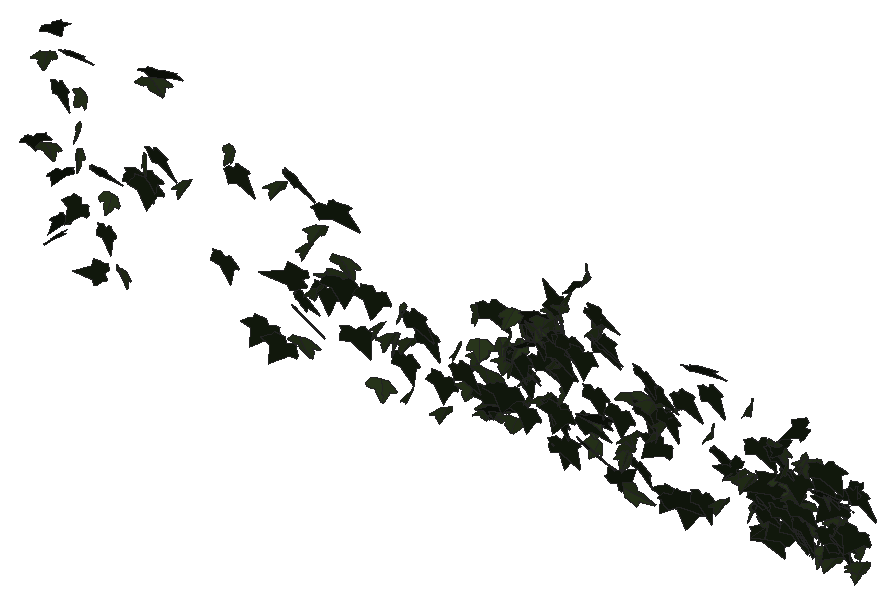
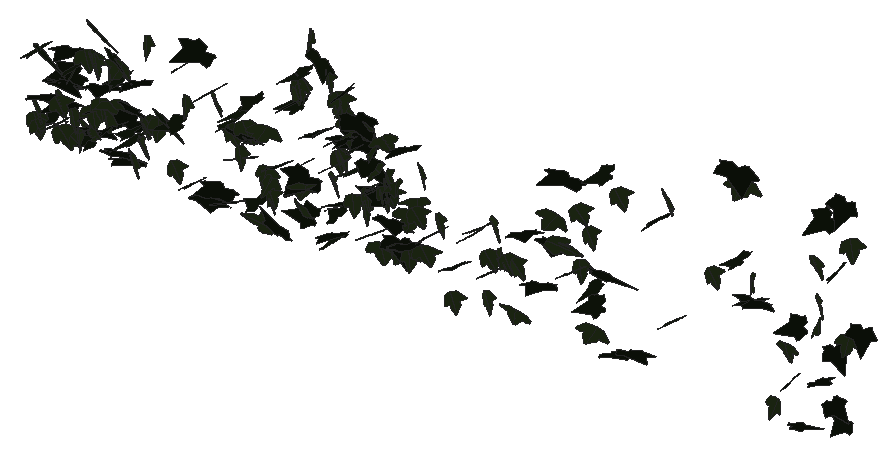
# SketchUp Ruby script. Lengths in millimetres.
U = 1.mm
M = Sketchup.active_model
def pt(a) = Geom::Point3d.new(a.map { |v| v * U })
def face(e, loops, mat)
  f = e.add_face(loops[0].map { |a| pt(a) })
  loops[1..].each { |l| e.add_face(l.map { |a| pt(a) }).erase! }
  f.material = f.back_material = mat if mat
  f
end
# faces: each face lists its corners as indices into pts; further lists are holes
def faces(e, pts, list, mat = nil) = list.each { |f| face(e, (f[0].is_a?(Array) ? f : [f]).map { |l| l.map { |i| pts[i] } }, mat) }
# xy, xz, yz: faces in a plane at the given z, y or x. An outline is a flat list of corners, or four numbers for a rectangle; further outlines are holes
def ring(l) = l.size == 4 ? [[l[0], l[1]], [l[2], l[1]], [l[2], l[3]], [l[0], l[3]]] : l.each_slice(2).to_a
def flat(e, list, mat, &to3) = list.each { |f| face(e, (f[0].is_a?(Array) ? f : [f]).map { |l| ring(l).map { |u, v| to3.(u, v) } }, mat) }
def xy(e, z, list, mat = nil) = flat(e, list, mat) { |x, y| [x, y, z] }
def xz(e, y, list, mat = nil) = flat(e, list, mat) { |x, z| [x, y, z] }
def yz(e, x, list, mat = nil) = flat(e, list, mat) { |y, z| [x, y, z] }
def lines(e, pts, list) = list.each { |a, b| e.add_line(pt(pts[a]), pt(pts[b])) }
# prism: a flat outline (further loops are holes) pulled along v
def prism(e, loops, v, mat = nil)
  f = face(e, loops, mat); d = Geom::Vector3d.new(v.map { |x| x * U })
  f.pushpull(f.normal.samedirection?(d) ? d.length : -d.length)
end
def box(e, o, s, mat = nil) = prism(e, [[o, [o[0] + s[0], o[1], o[2]], [o[0] + s[0], o[1] + s[1], o[2]], [o[0], o[1] + s[1], o[2]]]], [0, 0, s[2]], mat)
def at(x, y, z, deg = 0) = Geom::Transformation.translation(pt([x, y, z])) * Geom::Transformation.rotation(ORIGIN, Z_AXIS, deg.degrees)
def axes(o, x, y, z) = Geom::Transformation.new([*x, 0, *y, 0, *z, 0, *pt(o).to_a, 1])
def part(name) = M.definitions.add(name)
# library, detail: a bought-in or finely detailed component or shape, given as its bounding box
def library(name, o, s) = part(name).tap { |d| box(d.entities, o, s) }
def detail(e, o, s) = box(e.add_group.entities, o, s)
def put(e, d, t, mat = nil) = e.add_instance(d, t).tap { |i| i.material = mat if mat }
def group(e, t, mat = nil) = e.add_group.tap { |g| g.transformation = t; g.material = mat if mat }.entities
root = M.entities
M.materials.add("efeu1").color = [18, 25, 13]
M.materials.add("efeu2").color = [43, 57, 29]
c1 = part("ivyleaf_9")
p = [[39.1,54.8,31.7],[34.5,51.8,30.2],[-5.3,25.2,17.3],[-17.9,28.3,20.9],[-21.6,21.7,17],[-20.2,4.3,5.3],
  [-22.9,-0.3,2.5],[-17.1,-4,-0.6],[-2,-2.1,-1.2],[-0.7,-15.4,-10.1],[16.6,-22.3,-16.7],[21.1,-15.1,-12.5],
  [32.7,-10.7,-11],[46.1,-1.8,-6.6],[30.8,11.2,3.8]]
faces(c1.entities,p,[[0,1,2,3,4,5,6,7,8,9,10,11,12,13,14]],"efeu1")
c2 = part("ivyleaf_10")
p = [[0,12.8,-0.8],[-1.5,51.3,-10.9],[-4.9,51,-11.6],[-13.6,26.5,-7.3],[-13.2,15.9,-4.6],[-21.1,19.3,-7.2],
  [-29.5,16.3,-8.3],[-29.2,8.3,-6.2],[-19.7,-9.8,0.5],[-7.6,-13,4],[1,-12.2,5.8],[-0.4,51.1,-11.1],
  [-1.5,51.1,-10.9],[1,-12.4,5.9],[16.9,-12.4,3.5],[35.1,9.1,-5.1],[35,12.9,-6.1],[20.5,16.4,-4.9],
  [15.8,15,-3.8],[15.3,27.6,-7.1],[12.8,31.3,-7.8]]
faces(c2.entities,p,[[0,1,2,3,4,5,6,7,8,9,10],[11,12,0,13,14,15,16,17,18,19,20]],"efeu2")
put(root,c1,axes([498.7,807.1,3019.4],[0.64883,0.9298,-0.32357],[-0.16302,-0.29619,-1.07074],[-1.18997,0.54755,-0.02974]))
put(root,c2,axes([536.4,818.9,3310.7],[-0.85076,-0.89688,0.10443],[-0.07775,-0.08274,-1.13608],[1.09884,-0.70025,0.00047]))
put(root,c2,axes([534.9,833.7,2989],[-1.20869,-0.398,-0.15235],[0.16883,0.06422,-1.06766],[0.49175,-1.00032,-0.00792]))
put(root,c1,axes([565.2,809.5,2689.2],[0.52831,0.76397,0.62208],[0.16447,0.62718,-0.86407],[-1.19064,0.42562,0.15667]))
put(root,c1,axes([569.7,802.8,3431.6],[0.78365,0.97487,-0.01908],[-0.00827,-0.01839,-1.16745],[-1.18954,0.64236,-0.00445]))
put(root,c1,axes([583.9,843.7,2757.8],[-0.10885,0.66953,-0.82047],[0.03857,-0.82133,-0.67367],[-1.29139,-0.08097,0.04904]))
put(root,c1,axes([593.4,820.7,2929.5],[0.12701,0.93156,-0.55945],[-0.14034,-0.54941,-0.93624],[-1.31826,0.14824,0.04577]))
put(root,c1,axes([572.5,836.3,3210.3],[0.52799,-1.03242,0.01485],[0.01625,-0.01052,-1.11943],[1.25958,0.43291,0.00821]))
put(root,c1,axes([639.6,854.3,2815.3],[-0.77774,-0.81757,0.33916],[-0.10469,-0.35891,-1.02648],[1.07476,-0.62658,0.14544]))
put(root,c2,axes([648.1,835.7,3084.6],[0.66392,-0.9545,-0.19727],[-0.13784,0.16263,-1.0986],[1.18108,0.55553,-0.01732]))
put(root,c1,axes([631.7,804.9,3359.5],[1.39761,0.16278,0.1317],[0.1199,0.22876,-1.13763],[-0.22556,1.13021,0.21129]))
put(root,c2,axes([649,837.7,3000.5],[-0.19043,0.94722,-0.52335],[-0.00702,-0.52948,-0.95661],[-1.32025,-0.13381,0.08057]))
put(root,c2,axes([668.2,827.3,3212.4],[1.06368,-0.50726,-0.5025],[-0.4892,0.30837,-1.00702],[0.72076,0.9579,0.05809]))
put(root,c1,axes([738.2,836.1,2619.1],[-0.89773,0.10878,0.73853],[-0.89474,-0.29879,-0.68672],[0.16988,-0.99881,0.28586]))
put(root,c1,axes([712.8,835.4,2969.8],[1.23749,-0.20149,0.41978],[0.51766,-0.01439,-1.0322],[0.23393,1.09767,0.06353]))
put(root,c1,axes([748.9,842,2772.8],[0.23752,-1.05131,0.07293],[0.00124,-0.07398,-1.06911],[1.28568,0.1943,-0.01244]))
put(root,c2,axes([764.5,841.2,2887.6],[1.32303,-0.13951,-0.03035],[-0.03502,0.01473,-1.09333],[0.17063,1.08478,0.01095]))
put(root,c2,axes([825.7,821.4,2664.3],[-1.21327,0.54939,-0.06793],[0.08211,-0.01863,-1.13603],[-0.67035,-0.99662,-0.01621]))
put(root,c1,axes([885.1,847.2,3007.4],[-0.9972,-0.62003,-0.67499],[1.11767,0.36983,-0.79557],[1.33925,-0.77031,0.16135]))
put(root,c2,axes([897.1,839.8,3069.2],[0.6682,-0.97546,0.2369],[0.65545,-0.11869,-0.99911],[1.79451,0.40657,0.27671]))
put(root,c1,axes([914.3,838.4,2989.8],[-0.64593,-1.01454,0.0589],[0.03187,-0.06767,-1.06916],[1.93387,-0.33775,0.03729]))
put(root,c2,axes([954.1,812.9,3368.1],[-1.83481,-0.45281,-0.30173],[0.55191,0.09185,-1.06441],[0.87627,-1.00599,0.03863]))
put(root,c1,axes([977.2,809.9,3411.5],[1.19134,0.78464,-0.48189],[-0.79506,-0.27728,-0.99414],[-1.56174,0.73971,0.1385]))
put(root,c1,axes([949.4,827.6,3114.8],[0.88828,-0.98535,-0.02273],[0.07908,0.0448,-1.08882],[1.87415,0.46513,0.05671]))
put(root,c2,axes([1056.7,838.6,3040.1],[-0.25644,-1.03985,0.2075],[0.0435,-0.21196,-1.0474],[2.01758,-0.1276,0.04895]))
put(root,c1,axes([1195.2,854.8,2825.5],[-0.05206,-1.0253,0.17872],[0.05141,-0.17942,-1.02519],[1.98011,-0.0223,0.03131]))
put(root,c2,axes([1244.5,820.9,3225.3],[1.16075,-0.91075,-0.05301],[-0.02226,0.05595,-1.09589],[1.73614,0.60963,0.02139]))
put(root,c1,axes([1253.7,833,3157.9],[0.51408,-0.92167,-0.51108],[-0.19975,0.50145,-0.95977],[1.99578,0.2876,0.03559]))
put(root,c1,axes([1366.7,842.6,2657],[-1.55616,-0.66586,0.01126],[-0.01572,-0.00769,-1.05448],[1.26735,-0.8177,0.00074]))
put(root,c2,axes([1430.2,823.6,3174.2],[-0.53722,-1.01753,0.27722],[-0.06891,-0.27746,-1.05527],[2.00596,-0.28204,0.03799]))
put(root,c1,axes([1441,838.5,2623.7],[-1.25113,-0.79377,0.25529],[-0.22937,-0.23122,-1.02927],[1.57024,-0.66623,0.05306]))
put(root,c1,axes([1506.6,827,2872.8],[-1.48666,0.26971,0.6486],[-1.26477,0.03054,-0.81305],[-0.43316,-1.01486,0.1479]))
put(root,c1,axes([1469.3,819.3,3224.7],[1.4418,-0.77519,-0.19052],[-0.10821,0.20959,-1.07887],[1.51539,0.75251,0.10423]))
put(root,c1,axes([1509.3,815.2,2828.1],[1.44332,-0.50956,-0.60101],[-0.72181,0.49511,-0.89833],[1.31447,0.83138,0.16662]))
put(root,c2,axes([1522.3,821.8,2668.7],[-1.89549,0.08341,-0.22059],[0.40106,-0.11506,-0.99493],[-0.20152,-1.01357,0.09479]))
put(root,c1,axes([1498.3,825,2764.1],[1.61018,-0.67912,0.01835],[0.02902,-0.01032,-1.08489],[1.29265,0.84618,0.0015]))
put(root,c2,axes([1540.7,823.9,3001.8],[-0.14489,-1.0616,0.10446],[0.02964,-0.10582,-1.06408],[2.02998,-0.07423,0.02299]))
put(root,c2,axes([1576.9,832.4,3069.2],[-0.61036,-0.9462,0.41234],[-0.02787,-0.42757,-0.99254],[1.96418,-0.30009,0.11405]))
put(root,c2,axes([1580.5,814.7,2870.5],[-0.42398,-1.0028,-0.22556],[0.06314,0.22366,-1.02713],[1.9552,-0.22468,-0.01574]))
put(root,c1,axes([1590.6,851.2,2857.5],[-0.27523,-1.02549,0.18647],[-0.00253,-0.18807,-1.03535],[1.98372,-0.14252,0.02455]))
put(root,c2,axes([1662.1,836.9,2926.9],[0.58236,0.17713,-1.00278],[-1.93242,-0.02668,-0.31454],[-0.14761,1.04809,0.16147]))
put(root,c1,axes([1619.8,825.2,3163.6],[-0.20572,-0.35572,-1.02995],[1.06902,0.8687,-0.35898],[1.77705,-0.56377,0.09672]))
put(root,c1,axes([1666.6,831.8,2922.8],[-1.40357,-0.49811,-0.58047],[0.91574,0.3247,-0.88994],[1.13163,-0.88056,0.0002]))
put(root,c2,axes([1678.1,819.6,3002.1],[-1.91309,0.2156,-0.32106],[0.55471,-0.16535,-1.02357],[-0.48378,-1.04219,0.09598]))
put(root,c1,axes([1718,835.5,2765.3],[-0.51233,-0.81765,-0.59146],[0.46282,0.54154,-0.85932],[1.86401,-0.3592,0.0508]))
put(root,c1,axes([1787.3,837.9,2918.4],[-0.87006,-0.971,-0.0412],[0.00421,0.04449,-1.0731],[1.84967,-0.45685,-0.01694]))
put(root,c2,axes([1802.4,848.4,2809.7],[0.03678,-0.99801,0.34488],[0.01537,-0.34479,-0.9982],[2.00957,0.0209,0.00132]))
put(root,c2,axes([1820.2,823.7,2626.3],[1.90393,-0.09883,0.26611],[0.49748,-0.05949,-1.00473],[0.21071,1.03346,-0.03239]))
put(root,c2,axes([1856.5,825.2,2798.8],[-0.44814,-0.99051,0.24855],[0.03952,-0.25966,-1.01512],[1.94318,-0.22315,0.07796]))
put(root,c2,axes([1876.6,828.8,2800.7],[0.95621,-0.88255,0.4192],[0.44016,-0.35056,-1.01522],[1.80668,0.55251,0.02547]))
put(root,c2,axes([1902.6,829.3,2906.8],[0.69591,-1.00278,-0.06325],[-0.0284,0.06188,-1.06734],[1.91206,0.36588,0.00716]))
put(root,c2,axes([1916.7,841.7,2798.1],[-0.46992,-0.98046,0.29137],[-0.12193,-0.28433,-1.01105],[1.94284,-0.25499,0.00702]))
put(root,c1,axes([1907.6,834.2,2740.2],[0.00523,-1.03963,-0.01107],[0.00017,0.01107,-1.03963],[1.97873,0.00275,0.00012]))
put(root,c2,axes([1938.4,817.1,2638],[0.07579,-1.0123,-0.20358],[-0.04822,0.20271,-1.01294],[1.9646,0.04403,-0.01701]))
put(root,c1,axes([1927.7,840.4,2893.2],[0.63169,-0.96504,-0.31118],[0.10322,0.34386,-1.00852],[1.92702,0.29793,0.15603]))
put(root,c1,axes([1977.6,842.8,2845.4],[0.3758,-1.03466,-0.14421],[-0.01035,0.14574,-1.05311],[1.98817,0.19633,0.02178]))
put(root,c2,axes([2051.9,842.1,2606.9],[-0.54962,-0.98611,0.05415],[0.02446,-0.06016,-1.02711],[1.87943,-0.28759,0.0292]))
put(root,c1,axes([2048.8,841.5,2713.3],[-0.45637,-1.0029,0.13058],[-0.03273,-0.13014,-1.03108],[1.92454,-0.24003,0.01343]))
put(root,c2,axes([2113.4,829.2,2847.8],[0.30056,-1.0379,-0.15194],[-0.04649,0.14997,-1.04984],[1.99584,0.15979,-0.00157]))
put(root,c1,axes([2129.3,818.6,2792.9],[0.6445,-0.88892,-0.4643],[-0.11831,0.47051,-0.94615],[1.905,0.32996,0.09832]))
put(root,c2,axes([2163.6,842.6,2727.8],[-1.18737,-0.76186,0.3421],[-0.1166,-0.38412,-0.96716],[1.58516,-0.59893,0.18511]))
put(root,c2,axes([2183.6,828.9,2995.4],[0.88708,-0.89201,-0.40491],[-0.16422,0.40928,-1.00096],[1.85714,0.46226,0.10489]))
put(root,c2,axes([2192.7,844.8,2848.8],[-0.57845,-0.94095,0.36589],[-0.07103,-0.37137,-0.98606],[1.92012,-0.29721,0.07375]))
put(root,c2,axes([2190.4,836.4,2886.5],[1.1804,0.83815,-0.10849],[-0.11393,-0.09067,-1.04266],[-1.60443,0.62308,-0.00578]))
put(root,c2,axes([2231.3,822.7,2681.7],[-0.65199,-0.93883,-0.20194],[0.10087,0.1956,-0.99924],[1.82487,-0.34624,-0.01692]))
put(root,c2,axes([2236.3,818.4,2814.4],[-2.00001,0.04613,0.0573],[-0.10894,0.00251,-1.05188],[-0.08793,-1.05242,0]))
put(root,c1,axes([2225,847.6,2728.1],[-0.66583,-0.95472,-0.20152],[0.17461,0.18095,-1.01653],[1.84883,-0.36092,0.02343]))
put(root,c2,axes([2250.6,824.2,2692.2],[-1.69606,-0.4413,-0.29325],[0.53978,0.08738,-0.9934],[0.85177,-0.93409,0.04561]))
put(root,c1,axes([2274.6,815.3,2706.3],[0.66201,0.92965,-0.39975],[-0.27308,-0.37312,-0.99259],[-1.90649,0.37626,0.00337]))
put(root,c1,axes([2244.8,822.2,3043],[0.17914,-0.9504,-0.53101],[0.20808,0.53855,-0.94452],[2.06151,0.02823,0.14148]))
put(root,c2,axes([2271.2,840.8,2917.8],[0.2918,1.02837,-0.21556],[-0.22435,-0.19963,-1.03623],[-1.98711,0.17355,0.08534]))
put(root,c2,axes([2296.3,841.7,2934.5],[0.51526,-0.96086,0.35696],[0.37109,-0.31419,-0.9936],[1.91521,0.31938,0.09648]))
put(root,c2,axes([2311.6,830.2,2876],[-1.04338,-0.8563,0.28432],[-0.1071,-0.29959,-1.0108],[1.71385,-0.54003,0.10992]))
put(root,c1,axes([2302.5,829.1,2775.6],[-1.60874,-0.4313,-0.44212],[0.71447,0.23632,-0.94827],[0.93347,-0.92419,-0.03615]))
put(root,c2,axes([2309.9,836.5,2904.4],[0.37846,-1.04332,-0.15253],[0.11641,0.16638,-1.05826],[2.00338,0.18743,0.09031]))
put(root,c2,axes([2323,834.5,2864.5],[0.25671,-1.05588,-0.0346],[0.01521,0.0359,-1.06439],[2.01057,0.13454,0.01247]))
put(root,c2,axes([2328.2,824.7,3045.3],[1.01653,0.82489,-0.43726],[-0.68058,-0.28459,-0.97368],[-1.64136,0.62888,0.13292]))
put(root,c2,axes([2336.3,831.6,2675.4],[-1.69636,-0.47812,0.19014],[-0.29622,-0.11197,-1.01116],[0.9334,-0.90447,0.02466]))
put(root,c2,axes([2344.6,841,2939.1],[0.26895,0.795,-0.70096],[-0.44493,-0.66637,-0.8029],[-1.96751,0.25937,0.08575]))
put(root,c1,axes([2329,846.8,2886.5],[0.14882,-1.05398,0.07923],[0.01115,-0.07901,-1.05688],[2.01156,0.07841,0]))
put(root,c1,axes([2311.2,850.6,2859.3],[0.94413,-0.63665,0.68073],[0.77813,-0.54435,-0.80705],[1.5941,0.64278,-0.00923]))
put(root,c1,axes([2333.2,844.4,2898.7],[0.08691,-1.05775,0.09583],[-0.00557,-0.09605,-1.05871],[2.02135,0.04522,-0.00704]))
put(root,c1,axes([2376.3,838.7,2952.5],[-0.4674,0.82548,-0.63707],[-0.08416,-0.66216,-0.84094],[-1.98272,-0.16649,0.18587]))
put(root,c2,axes([2356.2,835,3009.8],[-0.34716,1.05483,0.06532],[-0.08361,0.05866,-1.06996],[-2.00965,-0.18466,0.03323]))
put(root,c1,axes([2362.1,851.5,2714],[-0.42331,-0.96615,0.28906],[0.07809,-0.30443,-0.98595],[1.91772,-0.20087,0.10396]))
put(root,c1,axes([2370.2,828.8,2859.9],[-0.04421,-1.05348,-0.00984],[0.00097,0.00983,-1.05373],[2.00507,-0.02323,0.00029]))
put(root,c2,axes([2390.3,827.1,2843],[-0.239,-1.04555,-0.18309],[0.06942,0.18001,-1.05297],[2.01898,-0.12996,0.01453]))
put(root,c2,axes([2397.1,828.2,2790.1],[0.24669,-1.02698,-0.23441],[0.07236,0.24058,-1.03301],[2.00352,0.11776,0.06617]))
put(root,c2,axes([2399.7,814,3032.1],[-1.67452,0.6414,0.04331],[-0.06208,0.02877,-1.0888],[-1.22191,-0.88044,-0.00403]))
put(root,c1,axes([2436.9,822,3079],[0.33889,0.76682,-0.74846],[-0.69142,-0.67059,-0.77346],[-1.91858,0.37711,0.14654]))
put(root,c1,axes([2403,837,3020.4],[-0.74008,-0.2086,-0.97796],[1.60849,0.49227,-0.44105],[1.01717,-0.93021,-0.0141]))
put(root,c1,axes([2415.2,838.7,2996.8],[0.08975,-1.01184,0.34823],[0.03727,-0.34769,-1.01293],[2.03624,0.05096,0.00319]))
put(root,c2,axes([2450,825.4,3060.7],[-1.92085,-0.36391,0.1748],[-0.27773,-0.11,-1.07155],[0.7164,-1.01837,0.05328]))
put(root,c2,axes([2446.7,825,2797.7],[-0.66412,-0.97798,-0.17168],[0.04775,0.17324,-1.03781],[1.88915,-0.34818,-0.03413]))
put(root,c1,axes([2417,840.3,2916.1],[0.84215,-0.89305,-0.33876],[0.09321,0.39407,-0.97488],[1.81543,0.39404,0.2072]))
put(root,c2,axes([2441,823.2,3020.7],[0.46762,1.05115,0.08164],[-0.18938,0.10658,-1.0727],[-1.99762,0.23596,0.12081]))
put(root,c1,axes([2438.7,843.6,3019.4],[0.17968,-0.96076,-0.45432],[0.10995,0.46007,-0.96092],[2.01966,0.06043,0.09273]))
put(root,c1,axes([2459.4,840.3,3009.1],[-0.79959,-0.8611,-0.47341],[0.48209,0.40257,-0.95703],[1.80699,-0.48843,0.04584]))
put(root,c2,axes([2492.6,826.4,2938],[0.22524,-1.06133,-0.04109],[-0.0442,0.03875,-1.06774],[2.02095,0.11913,-0.01877]))
put(root,c2,axes([2491.5,815,3082.1],[-0.28783,-0.99555,-0.3844],[0.12139,0.37911,-1.00696],[2.02744,-0.16403,0.00572]))
put(root,c1,axes([2503.5,822.5,3126.5],[-0.72891,-0.85783,0.56778],[0.4363,0.51945,0.93945],[-1.90862,0.44635,-0.00209]))
put(root,c1,axes([2481.5,854.2,2774.2],[-0.57221,-0.91202,0.39949],[-0.05988,-0.40839,-0.95603],[1.89402,-0.28845,0.09046]))
put(root,c2,axes([2498.3,837.4,2934],[-0.32893,-1.05243,0.04669],[0.05249,-0.05181,-1.06593],[2.00427,-0.17136,0.03558]))
put(root,c2,axes([2506.6,821,3127],[-0.90029,-0.98362,0.12394],[-0.01738,-0.13299,-1.09035],[1.88675,-0.47057,0.04909]))
put(root,c1,axes([2503.2,836.2,2767.3],[-0.8709,-0.91949,0.2445],[-0.02269,-0.26575,-1.0217],[1.81064,-0.4456,0.1048]))
put(root,c1,axes([2485.7,848.7,2735],[0.29047,-0.87701,0.5315],[0.17914,-0.52311,-0.89019],[1.94349,0.17929,0.00262]))
put(root,c2,axes([2502.9,825.8,3105.9],[-0.71814,0.88358,-0.52346],[0.31171,-0.49876,-0.95996],[-1.92957,-0.40942,0.03974]))
put(root,c1,axes([2502.9,851.5,2902.7],[-0.21839,-1.02273,0.2172],[-0.01377,-0.21772,-1.02901],[1.98982,-0.11375,0.01672]))
put(root,c1,axes([2495.7,824,2988.3],[0.36404,-1.03022,-0.24829],[0.06317,0.25801,-1.04495],[2.01587,0.17796,0.07758]))
put(root,c2,axes([2527.1,823.2,2840.1],[0.71188,-0.97216,-0.19561],[-0.15025,0.1792,-1.04159],[1.88131,0.38217,-0.00917]))
put(root,c1,axes([2510,853,2634],[-0.21933,-0.88068,0.49667],[-0.05664,-0.49672,-0.88767],[1.92346,-0.11505,0.0305]))
put(root,c1,axes([2508.1,839.5,2660.9],[0.00266,-0.92302,-0.46485],[0.26347,0.46082,-0.91462],[1.94916,-0.06103,0.12427]))
put(root,c2,axes([2548.3,815.6,3188.5],[0.2087,-1.05379,-0.32369],[0.00747,0.32566,-1.05887],[2.09805,0.10367,0.03597]))
put(root,c1,axes([2531,839.9,3016.5],[0.08543,-1.06825,-0.05661],[-0.00121,0.05664,-1.06919],[2.03594,0.04486,0.00174]))
put(root,c1,axes([2580.6,812.8,3228],[0.20297,0.98839,0.50155],[-0.07603,0.50697,-0.99057],[-2.10807,0.07688,0.08402]))
put(root,c1,axes([2581.8,843.8,2986.6],[-0.43687,-1.03616,0.0831],[-0.02632,-0.08205,-1.06127],[1.97818,-0.22992,0.00423]))
put(root,c2,axes([2623.6,805.7,3295.1],[0.36958,-0.8184,-0.74528],[0.14925,0.76493,-0.81955],[2.10135,0.08961,0.18929]))
put(root,c1,axes([2606.8,818,2782.5],[1.06131,-0.73407,-0.51362],[-0.08248,0.58218,-0.8791],[1.7031,0.48564,0.2775]))
put(root,c2,axes([2625,829.7,2779.9],[1.27374,0.82232,0.12267],[0.13212,0.10166,-1.0602],[-1.57684,0.67278,0.01026]))
put(root,c1,axes([2600.6,831.1,2683.9],[1.26105,-0.66477,0.49589],[0.65717,-0.35597,-0.93857],[1.43512,0.74714,-0.00595]))
put(root,c1,axes([2623,852.1,2867.5],[0.08597,-1.04483,0.03083],[0.00417,-0.03076,-1.04581],[1.98939,0.04521,0.00086]))
put(root,c2,axes([2644.1,829.2,2704.9],[1.52315,-0.67786,0.0243],[0.01791,-0.02648,-1.04871],[1.2908,0.80024,-0.01412]))
put(root,c1,axes([2631.5,811.7,2803.1],[1.80796,0.53749,0.09691],[0.16124,0.04706,-1.09147],[-1.02686,0.95373,-0.00076]))
put(root,c2,axes([2646.8,829,3135.7],[1.42946,-0.76225,-0.19976],[0.05877,0.30423,-1.04477],[1.49855,0.71518,0.23153]))
put(root,c2,axes([2657.5,831.8,3100.9],[-0.08954,-1.08106,0.03747],[0.00004,-0.0375,-1.08208],[2.0587,-0.04702,0.00165]))
put(root,c2,axes([2664.4,815.3,3115.5],[-0.50111,-1.01234,-0.29769],[0.091,0.29506,-1.04567],[2.00619,-0.26625,-0.02693]))
put(root,c1,axes([2634.9,818.2,3166],[1.35846,-0.70247,-0.44415],[-0.18195,0.51218,-0.96371],[1.57126,0.66664,0.2724]))
put(root,c1,axes([2639.5,836.3,3064.5],[1.26753,-0.84486,-0.05222],[0.09424,0.10522,-1.07077],[1.60825,0.6597,0.1039]))
put(root,c1,axes([2658.6,837.1,3063],[0.51509,-0.97158,-0.37476],[-0.02777,0.38363,-1.00512],[1.9817,0.25791,0.08332]))
put(root,c1,axes([2720.5,853.5,2828.3],[-0.39682,-1.01226,0.15527],[-0.004,-0.15804,-1.03309],[1.94906,-0.20642,0.02949]))
put(root,c1,axes([2720.8,840.1,2593.2],[-0.84911,0.5284,0.79464],[0.89576,-0.64124,0.69065],[1.57992,0.64754,0.03549]))
put(root,c2,axes([2753.2,833.3,2706.5],[-0.1366,-0.97612,0.28866],[0.33845,-0.29695,-0.95994],[1.90748,-0.01721,0.19099]))
put(root,c2,axes([2765.5,834.8,2697],[1.01412,-0.9002,0.0656],[0.03024,-0.06681,-1.04589],[1.71754,0.5327,-0.02032]))
put(root,c2,axes([2763.7,824.3,2749.8],[-0.46608,-0.78091,-0.68305],[0.46796,0.63814,-0.81772],[1.91829,-0.34541,0.03352]))
put(root,c2,axes([2781.6,825.5,2780.1],[-0.71282,-0.88638,-0.36893],[0.2274,0.3499,-0.96195],[1.81304,-0.39238,-0.0244]))
put(root,c2,axes([2783.5,830.2,2920.3],[-1.55576,-0.59294,-0.38587],[0.72076,0.13129,-1.00401],[1.13724,-0.89436,0.10844]))
put(root,c1,axes([2787.6,855.8,2672.8],[0.44978,-0.9186,0.42702],[0.27841,-0.40295,-0.94777],[1.90774,0.27538,0.03764]))
put(root,c2,axes([2777.7,824.2,2588.4],[-0.07605,-0.01063,1.12316],[2.13752,-0.01462,0.03982],[0.02709,1.12377,0.01114]))
put(root,c1,axes([2818,835.2,2891.7],[0.555,-1.00529,0.02952],[0.01647,-0.02823,-1.04673],[1.91402,0.29174,0.00044]))
put(root,c1,axes([2819.7,840.6,3002.4],[0.3195,-0.94714,0.47533],[0.25697,-0.45822,-0.96073],[2.00042,0.21014,0.0475]))
put(root,c2,axes([2855,837.6,2913.2],[-1.02907,-0.8953,0.20591],[-0.12199,-0.20159,-1.04479],[1.74416,-0.54233,0.04842]))
put(root,c1,axes([2864.5,852,2888.3],[-1.6171,-0.49482,-0.3867],[0.841,-0.00879,-0.95968],[0.84927,-0.93349,0.21402]))
put(root,c2,axes([2872.3,836.1,2818],[-0.02332,-1.03038,-0.27187],[0.088,0.27112,-1.02961],[2.02622,-0.02363,0.04159]))
put(root,c1,axes([2855.3,837.5,2962.9],[1.18709,-0.76712,-0.4187],[-0.1537,0.4616,-0.96604],[1.65618,0.59268,0.21046]))
put(root,c1,axes([2891,837.7,2787],[-1.30676,-0.62041,0.49026],[-0.27685,-0.5391,-0.88595],[1.47924,-0.64897,0.26728]))
put(root,c2,axes([2912.8,830.4,2874.8],[-0.28764,-1.04622,0.19358],[-0.04397,-0.19225,-1.05707],[2.02449,-0.15283,0.00454]))
put(root,c1,axes([2934.6,845.9,2621.5],[-1.15993,-0.73971,0.37944],[-0.1076,-0.43251,-0.93398],[1.57856,-0.57302,0.21515]))
put(root,c1,axes([2914.1,833.7,2897.7],[0.32426,-1.04692,0.13291],[0.05903,-0.1296,-1.06065],[2.00762,0.1729,0.00972]))
put(root,c2,axes([2964.5,842.3,2968.9],[1.06579,-0.9002,0.01051],[0.02793,-0.00324,-1.06011],[1.71314,0.56009,0.01075]))
put(root,c1,axes([2962.2,809.2,2646.1],[-0.01765,-0.23007,-1.06512],[0.7035,1.00134,-0.21951],[1.95092,-0.36316,0.06952]))
put(root,c1,axes([2975.9,823.2,2989.8],[0.73152,-0.88613,-0.4897],[-0.16659,0.49276,-0.96036],[1.91965,0.38044,0.10327]))
put(root,c1,axes([2995.2,842.5,2612.8],[-1.38924,-0.59799,-0.36276],[0.54271,0.22434,-0.9436],[1.21549,-0.78364,0.00669]))
put(root,c1,axes([3022.7,824.9,3103],[1.93183,0.24664,0.30481],[0.49967,0.20077,-1.03673],[-0.55427,1.04063,0.12778]))
put(root,c1,axes([3042.1,847.8,2654.7],[0.06477,-1.0252,-0.03651],[-0.01187,0.03632,-1.02575],[1.95236,0.03423,-0.00502]))
put(root,c2,axes([3094.8,817.8,2909],[-0.00618,-0.85845,-0.63854],[0.03595,0.63839,-0.85835],[2.03589,-0.01388,0.01322]))
put(root,c1,axes([3083.1,825.4,3045.6],[0.49528,-1.02512,-0.25312],[-0.1367,0.2429,-1.05759],[2.00494,0.26979,-0.00958]))
put(root,c2,axes([3130.2,830.5,2674.9],[-0.37991,-1.01518,0.1203],[-0.04169,-0.1183,-1.03462],[1.94516,-0.20081,0.00132]))
put(root,c1,axes([3102.9,838.2,2833.3],[1.42984,-0.75957,-0.11396],[0.10295,0.21134,-1.05203],[1.45817,0.72989,0.18602]))
put(root,c1,axes([3192.1,813.7,2815.3],[-0.93458,0.85867,0.33268],[-0.37588,0.27005,-0.98853],[-1.7118,-0.5281,0.03543]))
put(root,c2,axes([3195.5,823.2,2796.8],[-0.85008,-0.93006,-0.29734],[0.18139,0.28389,-1.03114],[1.84948,-0.45533,-0.03554]))
put(root,c2,axes([3232.5,828.3,2789.7],[-0.30792,-0.97806,0.34417],[-0.02844,-0.3461,-0.99056],[1.97312,-0.15762,0.03943]))
put(root,c2,axes([3235.4,845,2785.6],[1.11406,-0.83707,0.25306],[0.29821,-0.1992,-1.02134],[1.63739,0.60581,0.01383]))
put(root,c2,axes([3250.6,811.3,3055.8],[0.14615,-0.99229,-0.44675],[0.15149,0.45178,-0.98979],[2.06556,0.03708,0.1042]))
put(root,c2,axes([3257.2,827.5,2704.5],[0.85988,-0.92911,0.29151],[0.17292,-0.27974,-1.0324],[1.84519,0.45919,-0.0391]))
put(root,c2,axes([3289.2,834.6,2654.2],[1.11967,-0.94171,-0.38932],[-0.23178,0.38135,-1.10646],[1.92549,0.59351,0.0932]))
put(root,c1,axes([3265.1,838.7,2919.7],[-0.0821,-0.93139,-0.50119],[0.30663,0.48997,-0.9244],[1.98948,-0.11395,0.12179]))
put(root,c1,axes([3279.3,822.5,2713.6],[1.24281,-0.72226,-0.52996],[-0.2766,0.56171,-0.94461],[1.68235,0.62591,0.23619]))
put(root,c1,axes([3280.9,838.2,2742.9],[0.70725,-0.96197,0.06849],[0.10103,-0.05289,-1.0308],[1.83267,0.37415,0.03039]))
put(root,c1,axes([3340.4,825.4,2809.7],[-1.90957,0.05538,0.27568],[-0.52931,-0.04482,-1.0032],[-0.07891,-1.03956,0.05794]))
put(root,c1,axes([3299.2,832.8,2633.3],[-0.39292,-0.83999,-0.54914],[0.88816,0.41598,-0.81175],[1.69091,-0.41368,0.29877]))
put(root,c1,axes([3293.6,816,2767.5],[0.49863,-0.23663,-1.0328],[1.22834,0.8794,-0.03776],[1.59928,-0.60165,0.35101]))
put(root,c1,axes([3366.7,842,2645.9],[-1.75167,-0.13165,0.44521],[-0.77358,-0.24917,-0.91397],[0.42696,-0.99158,0.17056]))
put(root,c1,axes([3320.4,839.6,2912.1],[0.84516,-0.96053,-0.05264],[0.02507,0.06405,-1.0575],[1.83065,0.44257,0.03879]))
put(root,c2,axes([3343,827.9,2943.5],[-1.78587,0.47195,-0.16449],[0.23268,-0.12253,-1.04897],[-0.92231,-0.94475,0.05388]))
put(root,c1,axes([3377.9,810.3,2955.9],[-0.73471,0.9338,0.36352],[-0.22457,0.34449,-1.01023],[-1.89386,-0.40311,-0.02123]))
put(root,c2,axes([3358.8,842.6,2814.4],[1.35231,0.66056,-0.44439],[-0.6401,-0.29082,-0.97006],[-1.37335,0.78599,0.01455]))
put(root,c1,axes([3354.2,835.8,2734.3],[0.21869,-0.97087,-0.37461],[0.0161,0.37775,-0.97641],[1.98048,0.10414,0.0493]))
put(root,c2,axes([3380.5,839.7,2769.4],[1.46476,-0.73395,-0.13089],[0.10217,0.24219,-1.0424],[1.4152,0.74217,0.21072]))
put(root,c2,axes([3389.8,812.4,2900],[0.41207,-0.95794,-0.47403],[0.09934,0.49256,-0.97155],[2.03173,0.1702,0.14365]))
put(root,c2,axes([3413.6,832.9,2792.1],[-0.79242,-0.95888,-0.06122],[0.01876,0.06246,-1.04525],[1.82855,-0.41618,-0.01581]))
put(root,c1,axes([3408.4,836.4,2855.8],[-0.84395,-0.91696,-0.33872],[0.2749,0.30639,-1.01855],[1.84,-0.46636,-0.00318]))
put(root,c1,axes([3445.6,828.1,3041],[-1.71067,0.55758,-0.22216],[0.3002,-0.16655,-1.05619],[-1.10216,-0.91078,0.05714]))
put(root,c2,axes([3434,840.4,2763.1],[-1.35487,-0.77935,0.03393],[0.06242,-0.07579,-1.05286],[1.48335,-0.70866,0.07529]))
put(root,c2,axes([3440,818.9,2927.7],[0.06624,-1.02892,-0.38326],[-0.03761,0.3828,-1.02949],[2.08933,0.03951,-0.00638]))
put(root,c1,axes([3418.9,830.3,2771.1],[0.46187,-0.87891,-0.54607],[-0.02649,0.55806,-0.9044],[1.96912,0.21366,0.11591]))
put(root,c1,axes([3426,834.3,2692.8],[-0.96468,-0.74297,-0.51958],[0.92319,0.28066,-0.87454],[1.45775,-0.66941,0.21001]))
put(root,c2,axes([3451.9,825,2933.7],[0.74136,-1.0206,-0.04743],[0.0171,0.05417,-1.09206],[1.94443,0.38865,0.02768]))
put(root,c2,axes([3451.7,840.5,2698.9],[1.64501,-0.57614,0.0617],[0.10442,-0.02894,-1.03874],[1.09783,0.86606,0.00634]))
put(root,c1,axes([3432,836.7,2658.1],[0.91933,-0.90652,0.15769],[0.12879,-0.14261,-1.02716],[1.74646,0.48771,-0.00726]))
put(root,c1,axes([3439.5,832.8,2706.1],[0.26079,-1.05273,0.13672],[0.02547,-0.13613,-1.06161],[2.02023,0.13761,-0.00426]))
put(root,c2,axes([3475.1,825.2,2934.1],[-1.10036,-0.91228,0.16133],[0.06826,-0.21206,-1.07065],[1.76187,-0.56154,0.14223]))
put(root,c1,axes([3455.9,840.6,2655.5],[0.00528,-0.77898,0.71508],[0.08768,-0.71431,-0.77832],[2.01058,0.0332,0.03206]))
put(root,c2,axes([3495.6,827.8,2656.8],[0.09421,-0.82381,-0.61806],[-0.07184,0.6169,-0.82529],[1.95875,0.06225,-0.00054]))
put(root,c2,axes([3514.6,835.7,2721.6],[0.08347,-1.04284,-0.2309],[0.0018,0.23114,-1.04371],[2.0328,0.04262,0.0104]))
put(root,c2,axes([3514.7,834.8,2636.9],[-0.24206,-0.77001,0.67294],[0.48235,-0.68071,-0.73099],[1.88555,0.07528,0.27339]))
put(root,c1,axes([3510.1,832.7,2881.3],[0.65545,-1.00501,-0.12122],[0.00923,0.12968,-1.06137],[1.92658,0.3413,0.04633]))
put(root,c2,axes([3532.6,814.9,2856.3],[-0.64954,1.00124,-0.06655],[0.04307,-0.06259,-1.05781],[-1.90928,-0.34204,-0.00122]))
put(root,c1,axes([3528.3,827.8,2935.2],[-0.49787,-0.79135,-0.69858],[0.57704,0.63305,-0.83066],[1.92432,-0.39457,0.06835]))
put(root,c1,axes([3563.2,840,2816.7],[-1.85218,-0.41909,-0.03941],[0.06405,0.0215,-1.05957],[0.79856,-0.97375,-0.00643]))
put(root,c1,axes([3519.1,812.9,2847.4],[1.97036,-0.06916,0.21352],[0.41742,0.09786,-1.03175],[0.09066,1.05254,0.10996]))
put(root,c2,axes([3566.7,825.6,2640.3],[-0.73504,-1.05676,0.39393],[-0.18069,-0.38444,-1.12439],[2.13879,-0.39565,0.04039]))
put(root,c2,axes([3565.9,845.5,2750.6],[-0.67517,-0.93148,0.34824],[0.04414,-0.37739,-0.98581],[1.89211,-0.32358,0.14726]))
put(root,c1,axes([3569.3,843,2673.6],[-1.19907,-0.67663,0.47075],[-0.16004,-0.53666,-0.88391],[1.56058,-0.57492,0.27105]))
put(root,c1,axes([3545.8,840.3,2689.3],[0.78888,-0.89348,-0.41572],[-0.07699,0.43519,-0.97566],[1.87395,0.39401,0.13492]))
put(root,c2,axes([3578.4,826.3,2756.1],[0.53186,-1.01362,-0.26101],[-0.06123,0.2617,-1.05077],[1.9911,0.2788,0.03741]))
put(root,c1,axes([3555.5,815.9,2733.8],[0.17804,-0.6302,-0.83409],[0.41983,0.83046,-0.60273],[1.9448,-0.12158,0.20647]))
put(root,c1,axes([3570.5,838,2697.1],[0.3835,-0.94978,0.45185],[0.16653,-0.44334,-0.97091],[1.99483,0.2196,-0.00582]))
put(root,c1,axes([3650.3,827.1,2892],[-1.40962,0.78649,0.00398],[-0.02291,-0.00588,-1.08027],[-1.4967,-0.74065,0.01279]))
put(root,c1,axes([3639.9,840.7,2741.1],[-1.16793,-0.82906,0.1765],[-0.0945,-0.18236,-1.02925],[1.61046,-0.61195,0.0676]))
put(root,c2,axes([3660.7,828,2632.6],[-0.5573,-0.95672,0.26524],[0.1828,-0.30254,-0.98522],[1.88065,-0.2541,0.17437]))
put(root,c2,axes([3667.3,827.2,2701.7],[0.85296,-0.86397,-0.43718],[-0.27804,0.41589,-0.97166],[1.82175,0.468,0.05639]))
put(root,c2,axes([3670.9,822.2,2650.1],[-0.76981,-0.93336,0.14182],[-0.05549,-0.14186,-1.01681],[1.79589,-0.40447,0.02937]))
put(root,c1,axes([3651.1,821.6,2892.1],[0.74471,-0.98507,-0.26716],[-0.06482,0.27336,-1.05781],[1.94144,0.38699,0.06716]))
